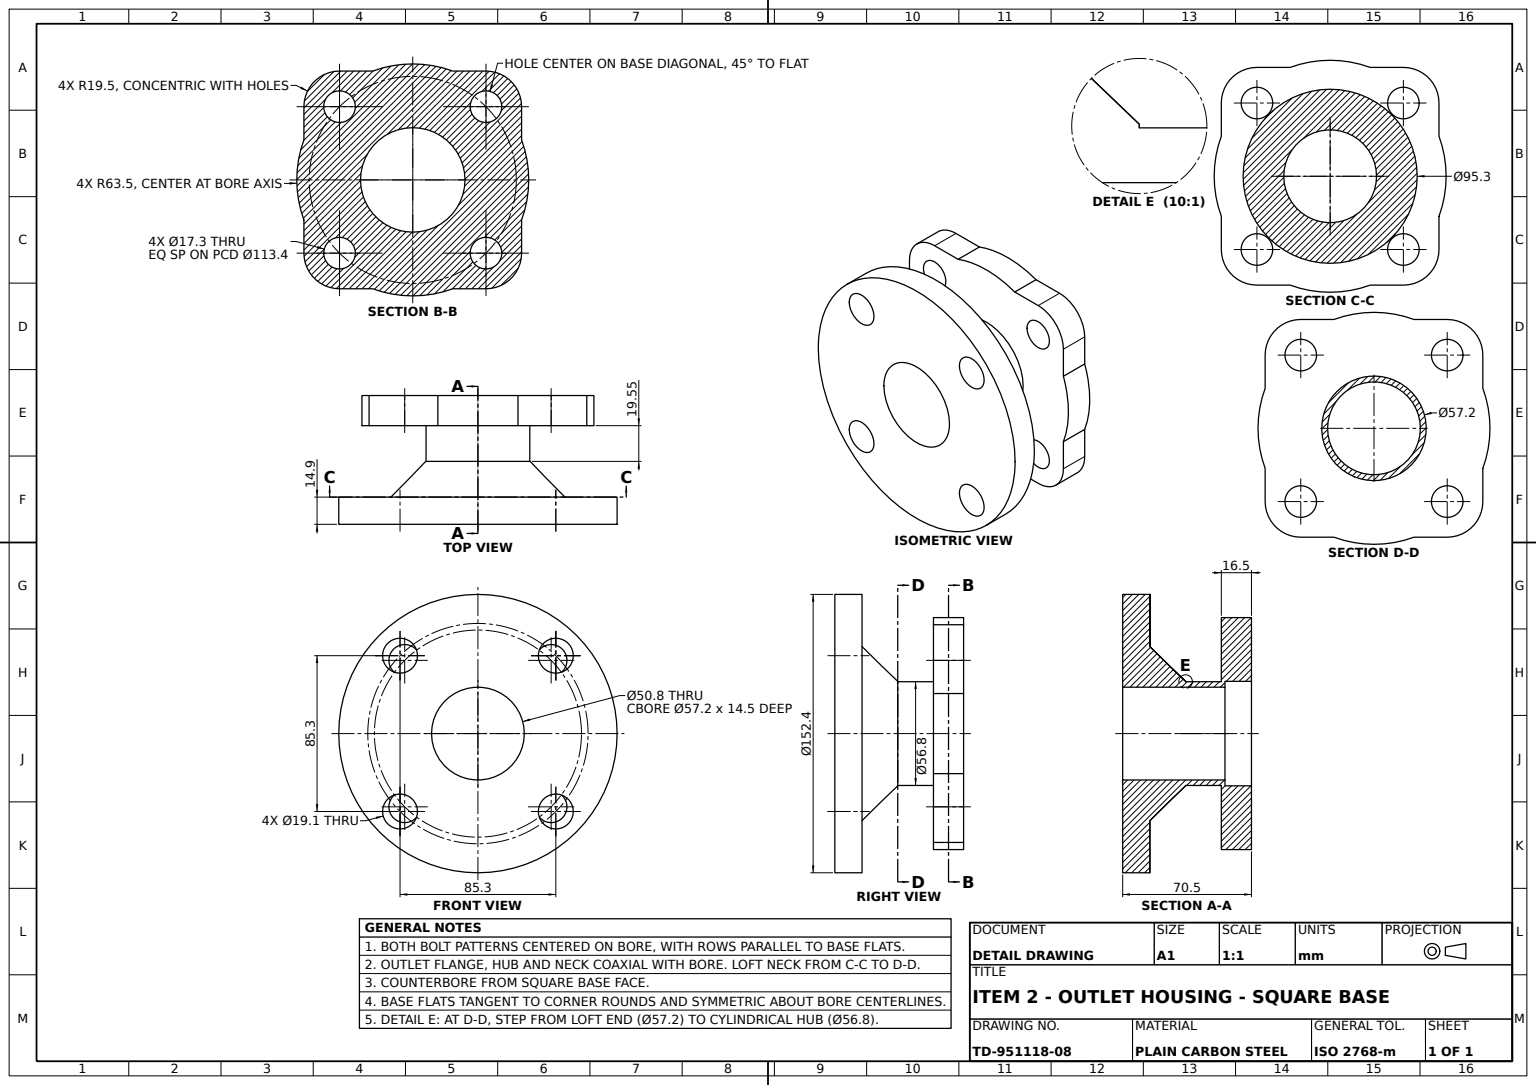
ISO-10303-21;
HEADER;
FILE_DESCRIPTION((''),'2;1');
FILE_NAME('','',(''),(''),'','','');
FILE_SCHEMA(('AUTOMOTIVE_DESIGN'));
ENDSEC;
DATA;
#1=APPLICATION_CONTEXT('');
#2=PRODUCT_CONTEXT('',#1,'mechanical');
#3=PRODUCT('','','',(#2));
#4=PRODUCT_DEFINITION_FORMATION('','',#3);
#5=PRODUCT_DEFINITION_CONTEXT('',#1,'design');
#6=PRODUCT_DEFINITION('','',#4,#5);
#7=PRODUCT_DEFINITION_SHAPE('','',#6);
#8=(LENGTH_UNIT()NAMED_UNIT(*)SI_UNIT(.MILLI.,.METRE.));
#9=(NAMED_UNIT(*)PLANE_ANGLE_UNIT()SI_UNIT($,.RADIAN.));
#10=(NAMED_UNIT(*)SI_UNIT($,.STERADIAN.)SOLID_ANGLE_UNIT());
#11=UNCERTAINTY_MEASURE_WITH_UNIT(LENGTH_MEASURE(1.E-05),#8,'distance_accuracy_value','');
#12=(GEOMETRIC_REPRESENTATION_CONTEXT(3)GLOBAL_UNCERTAINTY_ASSIGNED_CONTEXT((#11))GLOBAL_UNIT_ASSIGNED_CONTEXT((#8,#9,#10))REPRESENTATION_CONTEXT('',''));
#13=CARTESIAN_POINT('',(48.742954,40.092954,16.5));
#14=VERTEX_POINT('',#13);
#15=CARTESIAN_POINT('',(31.442954,40.092954,16.5));
#16=VERTEX_POINT('',#15);
#17=CARTESIAN_POINT('',(40.092954,40.092954,16.5));
#18=DIRECTION('',(0.,0.,1.));
#19=DIRECTION('',(1.,0.,0.));
#20=AXIS2_PLACEMENT_3D('',#17,#18,#19);
#21=CIRCLE('',#20,8.65);
#22=EDGE_CURVE('',#14,#16,#21,.T.);
#23=ORIENTED_EDGE('',*,*,#22,.F.);
#24=EDGE_CURVE('',#16,#14,#21,.T.);
#25=ORIENTED_EDGE('',*,*,#24,.F.);
#26=EDGE_LOOP('',(#23,#25));
#27=FACE_BOUND('',#26,.T.);
#28=CARTESIAN_POINT('',(-31.442954,-40.092954,16.5));
#29=VERTEX_POINT('',#28);
#30=CARTESIAN_POINT('',(-48.742954,-40.092954,16.5));
#31=VERTEX_POINT('',#30);
#32=CARTESIAN_POINT('',(-40.092954,-40.092954,16.5));
#33=AXIS2_PLACEMENT_3D('',#32,#18,#19);
#34=CIRCLE('',#33,8.65);
#35=EDGE_CURVE('',#29,#31,#34,.T.);
#36=ORIENTED_EDGE('',*,*,#35,.F.);
#37=EDGE_CURVE('',#31,#29,#34,.T.);
#38=ORIENTED_EDGE('',*,*,#37,.F.);
#39=EDGE_LOOP('',(#36,#38));
#40=FACE_BOUND('',#39,.T.);
#41=CARTESIAN_POINT('',(-48.742954,40.092954,16.5));
#42=VERTEX_POINT('',#41);
#43=CARTESIAN_POINT('',(-31.442954,40.092954,16.5));
#44=VERTEX_POINT('',#43);
#45=CARTESIAN_POINT('',(-40.092954,40.092954,16.5));
#46=AXIS2_PLACEMENT_3D('',#45,#18,#19);
#47=CIRCLE('',#46,8.65);
#48=EDGE_CURVE('',#42,#44,#47,.T.);
#49=ORIENTED_EDGE('',*,*,#48,.F.);
#50=EDGE_CURVE('',#44,#42,#47,.T.);
#51=ORIENTED_EDGE('',*,*,#50,.F.);
#52=EDGE_LOOP('',(#49,#51));
#53=FACE_BOUND('',#52,.T.);
#54=CARTESIAN_POINT('',(48.742954,-40.092954,16.5));
#55=VERTEX_POINT('',#54);
#56=CARTESIAN_POINT('',(31.442954,-40.092954,16.5));
#57=VERTEX_POINT('',#56);
#58=CARTESIAN_POINT('',(40.092954,-40.092954,16.5));
#59=AXIS2_PLACEMENT_3D('',#58,#18,#19);
#60=CIRCLE('',#59,8.65);
#61=EDGE_CURVE('',#55,#57,#60,.T.);
#62=ORIENTED_EDGE('',*,*,#61,.F.);
#63=EDGE_CURVE('',#57,#55,#60,.T.);
#64=ORIENTED_EDGE('',*,*,#63,.F.);
#65=EDGE_LOOP('',(#62,#64));
#66=FACE_BOUND('',#65,.T.);
#67=CARTESIAN_POINT('',(59.592954,-21.930111,16.5));
#68=VERTEX_POINT('',#67);
#69=CARTESIAN_POINT('',(59.592954,21.930111,16.5));
#70=VERTEX_POINT('',#69);
#71=CARTESIAN_POINT('',(0.,0.,16.5));
#72=AXIS2_PLACEMENT_3D('',#71,#18,#19);
#73=CIRCLE('',#72,63.5);
#74=EDGE_CURVE('',#68,#70,#73,.T.);
#75=ORIENTED_EDGE('',*,*,#74,.T.);
#76=CARTESIAN_POINT('',(59.592954,40.092954,16.5));
#77=VERTEX_POINT('',#76);
#78=CARTESIAN_POINT('',(59.592954,0.,16.5));
#79=DIRECTION('',(0.,1.,0.));
#80=VECTOR('',#79,1000.);
#81=LINE('',#78,#80);
#82=EDGE_CURVE('',#70,#77,#81,.T.);
#83=ORIENTED_EDGE('',*,*,#82,.T.);
#84=CARTESIAN_POINT('',(40.092954,59.592954,16.5));
#85=VERTEX_POINT('',#84);
#86=CIRCLE('',#20,19.5);
#87=EDGE_CURVE('',#77,#85,#86,.T.);
#88=ORIENTED_EDGE('',*,*,#87,.T.);
#89=CARTESIAN_POINT('',(21.930111,59.592954,16.5));
#90=VERTEX_POINT('',#89);
#91=CARTESIAN_POINT('',(0.,59.592954,16.5));
#92=VECTOR('',#19,1000.);
#93=LINE('',#91,#92);
#94=EDGE_CURVE('',#90,#85,#93,.T.);
#95=ORIENTED_EDGE('',*,*,#94,.F.);
#96=CARTESIAN_POINT('',(-21.930111,59.592954,16.5));
#97=VERTEX_POINT('',#96);
#98=EDGE_CURVE('',#90,#97,#73,.T.);
#99=ORIENTED_EDGE('',*,*,#98,.T.);
#100=CARTESIAN_POINT('',(-40.092954,59.592954,16.5));
#101=VERTEX_POINT('',#100);
#102=EDGE_CURVE('',#101,#97,#93,.T.);
#103=ORIENTED_EDGE('',*,*,#102,.F.);
#104=CARTESIAN_POINT('',(-59.592954,40.092954,16.5));
#105=VERTEX_POINT('',#104);
#106=DIRECTION('',(0.,0.,-1.));
#107=AXIS2_PLACEMENT_3D('',#45,#106,#19);
#108=CIRCLE('',#107,19.5);
#109=EDGE_CURVE('',#105,#101,#108,.T.);
#110=ORIENTED_EDGE('',*,*,#109,.F.);
#111=CARTESIAN_POINT('',(-59.592954,21.930111,16.5));
#112=VERTEX_POINT('',#111);
#113=CARTESIAN_POINT('',(-59.592954,0.,16.5));
#114=LINE('',#113,#80);
#115=EDGE_CURVE('',#112,#105,#114,.T.);
#116=ORIENTED_EDGE('',*,*,#115,.F.);
#117=CARTESIAN_POINT('',(-63.5,0.,16.5));
#118=VERTEX_POINT('',#117);
#119=EDGE_CURVE('',#112,#118,#73,.T.);
#120=ORIENTED_EDGE('',*,*,#119,.T.);
#121=CARTESIAN_POINT('',(-59.592954,-21.930111,16.5));
#122=VERTEX_POINT('',#121);
#123=EDGE_CURVE('',#118,#122,#73,.T.);
#124=ORIENTED_EDGE('',*,*,#123,.T.);
#125=CARTESIAN_POINT('',(-59.592954,-40.092954,16.5));
#126=VERTEX_POINT('',#125);
#127=EDGE_CURVE('',#126,#122,#114,.T.);
#128=ORIENTED_EDGE('',*,*,#127,.F.);
#129=CARTESIAN_POINT('',(-40.092954,-59.592954,16.5));
#130=VERTEX_POINT('',#129);
#131=CIRCLE('',#33,19.5);
#132=EDGE_CURVE('',#126,#130,#131,.T.);
#133=ORIENTED_EDGE('',*,*,#132,.T.);
#134=CARTESIAN_POINT('',(-21.930111,-59.592954,16.5));
#135=VERTEX_POINT('',#134);
#136=CARTESIAN_POINT('',(0.,-59.592954,16.5));
#137=DIRECTION('',(-1.,0.,0.));
#138=VECTOR('',#137,1000.);
#139=LINE('',#136,#138);
#140=EDGE_CURVE('',#135,#130,#139,.T.);
#141=ORIENTED_EDGE('',*,*,#140,.F.);
#142=CARTESIAN_POINT('',(21.930111,-59.592954,16.5));
#143=VERTEX_POINT('',#142);
#144=EDGE_CURVE('',#135,#143,#73,.T.);
#145=ORIENTED_EDGE('',*,*,#144,.T.);
#146=CARTESIAN_POINT('',(40.092954,-59.592954,16.5));
#147=VERTEX_POINT('',#146);
#148=EDGE_CURVE('',#147,#143,#139,.T.);
#149=ORIENTED_EDGE('',*,*,#148,.F.);
#150=CARTESIAN_POINT('',(59.592954,-40.092954,16.5));
#151=VERTEX_POINT('',#150);
#152=AXIS2_PLACEMENT_3D('',#58,#106,#19);
#153=CIRCLE('',#152,19.5);
#154=EDGE_CURVE('',#151,#147,#153,.T.);
#155=ORIENTED_EDGE('',*,*,#154,.F.);
#156=DIRECTION('',(0.,-1.,0.));
#157=VECTOR('',#156,1000.);
#158=LINE('',#78,#157);
#159=EDGE_CURVE('',#68,#151,#158,.T.);
#160=ORIENTED_EDGE('',*,*,#159,.F.);
#161=EDGE_LOOP('',(#75,#83,#88,#95,#99,#103,#110,#116,#120,#124,#128,#133,#141,#145,#149,#155,#160));
#162=FACE_OUTER_BOUND('',#161,.T.);
#163=CARTESIAN_POINT('',(-28.4,0.,16.5));
#164=VERTEX_POINT('',#163);
#165=CARTESIAN_POINT('',(28.4,0.,16.5));
#166=VERTEX_POINT('',#165);
#167=CIRCLE('',#72,28.4);
#168=EDGE_CURVE('',#164,#166,#167,.T.);
#169=ORIENTED_EDGE('',*,*,#168,.F.);
#170=EDGE_CURVE('',#166,#164,#167,.T.);
#171=ORIENTED_EDGE('',*,*,#170,.F.);
#172=EDGE_LOOP('',(#169,#171));
#173=FACE_BOUND('',#172,.T.);
#174=PLANE('',#72);
#175=ADVANCED_FACE('',(#27,#40,#53,#66,#162,#173),#174,.T.);
#176=CARTESIAN_POINT('',(-25.4,0.,14.5));
#177=VERTEX_POINT('',#176);
#178=CARTESIAN_POINT('',(25.4,0.,14.5));
#179=VERTEX_POINT('',#178);
#180=CARTESIAN_POINT('',(0.,0.,14.5));
#181=AXIS2_PLACEMENT_3D('',#180,#106,#137);
#182=CIRCLE('',#181,25.4);
#183=EDGE_CURVE('',#177,#179,#182,.T.);
#184=ORIENTED_EDGE('',*,*,#183,.F.);
#185=EDGE_CURVE('',#179,#177,#182,.T.);
#186=ORIENTED_EDGE('',*,*,#185,.F.);
#187=EDGE_LOOP('',(#184,#186));
#188=FACE_BOUND('',#187,.T.);
#189=CARTESIAN_POINT('',(-28.6,0.,14.5));
#190=VERTEX_POINT('',#189);
#191=CARTESIAN_POINT('',(28.6,0.,14.5));
#192=VERTEX_POINT('',#191);
#193=CIRCLE('',#181,28.6);
#194=EDGE_CURVE('',#190,#192,#193,.T.);
#195=ORIENTED_EDGE('',*,*,#194,.T.);
#196=EDGE_CURVE('',#192,#190,#193,.T.);
#197=ORIENTED_EDGE('',*,*,#196,.T.);
#198=EDGE_LOOP('',(#195,#197));
#199=FACE_OUTER_BOUND('',#198,.T.);
#200=PLANE('',#181);
#201=ADVANCED_FACE('',(#188,#199),#200,.T.);
#202=CARTESIAN_POINT('',(-31.442954,40.092954,0.));
#203=VERTEX_POINT('',#202);
#204=CARTESIAN_POINT('',(-31.442954,40.092954,43.5));
#205=VECTOR('',#106,1000.);
#206=LINE('',#204,#205);
#207=EDGE_CURVE('',#44,#203,#206,.T.);
#208=ORIENTED_EDGE('',*,*,#207,.T.);
#209=CARTESIAN_POINT('',(-48.742954,40.092954,0.));
#210=VERTEX_POINT('',#209);
#211=CARTESIAN_POINT('',(-40.092954,40.092954,0.));
#212=AXIS2_PLACEMENT_3D('',#211,#106,#137);
#213=CIRCLE('',#212,8.65);
#214=EDGE_CURVE('',#203,#210,#213,.T.);
#215=ORIENTED_EDGE('',*,*,#214,.T.);
#216=CARTESIAN_POINT('',(-48.742954,40.092954,43.5));
#217=LINE('',#216,#205);
#218=EDGE_CURVE('',#42,#210,#217,.T.);
#219=ORIENTED_EDGE('',*,*,#218,.F.);
#220=ORIENTED_EDGE('',*,*,#48,.T.);
#221=EDGE_LOOP('',(#208,#215,#219,#220));
#222=FACE_OUTER_BOUND('',#221,.T.);
#223=CARTESIAN_POINT('',(-40.092954,40.092954,43.5));
#224=AXIS2_PLACEMENT_3D('',#223,#106,#137);
#225=CYLINDRICAL_SURFACE('',#224,8.65);
#226=ADVANCED_FACE('',(#222),#225,.F.);
#227=CARTESIAN_POINT('',(25.4,0.,70.5));
#228=VERTEX_POINT('',#227);
#229=CARTESIAN_POINT('',(-25.4,0.,70.5));
#230=VERTEX_POINT('',#229);
#231=CARTESIAN_POINT('',(0.,0.,70.5));
#232=AXIS2_PLACEMENT_3D('',#231,#18,#19);
#233=CIRCLE('',#232,25.4);
#234=EDGE_CURVE('',#228,#230,#233,.T.);
#235=ORIENTED_EDGE('',*,*,#234,.T.);
#236=CARTESIAN_POINT('',(-25.4,0.,109.9));
#237=LINE('',#236,#205);
#238=EDGE_CURVE('',#230,#177,#237,.T.);
#239=ORIENTED_EDGE('',*,*,#238,.T.);
#240=ORIENTED_EDGE('',*,*,#183,.T.);
#241=CARTESIAN_POINT('',(25.4,0.,109.9));
#242=LINE('',#241,#205);
#243=EDGE_CURVE('',#228,#179,#242,.T.);
#244=ORIENTED_EDGE('',*,*,#243,.F.);
#245=EDGE_LOOP('',(#235,#239,#240,#244));
#246=FACE_OUTER_BOUND('',#245,.T.);
#247=CARTESIAN_POINT('',(0.,0.,109.9));
#248=AXIS2_PLACEMENT_3D('',#247,#106,#137);
#249=CYLINDRICAL_SURFACE('',#248,25.4);
#250=ADVANCED_FACE('',(#246),#249,.F.);
#251=CARTESIAN_POINT('',(-40.092954,-59.592954,0.));
#252=VERTEX_POINT('',#251);
#253=LINE('',#129,#205);
#254=EDGE_CURVE('',#130,#252,#253,.T.);
#255=ORIENTED_EDGE('',*,*,#254,.T.);
#256=CARTESIAN_POINT('',(-21.930111,-59.592954,0.));
#257=VERTEX_POINT('',#256);
#258=CARTESIAN_POINT('',(0.,-59.592954,0.));
#259=LINE('',#258,#138);
#260=EDGE_CURVE('',#257,#252,#259,.T.);
#261=ORIENTED_EDGE('',*,*,#260,.F.);
#262=LINE('',#134,#205);
#263=EDGE_CURVE('',#135,#257,#262,.T.);
#264=ORIENTED_EDGE('',*,*,#263,.F.);
#265=ORIENTED_EDGE('',*,*,#140,.T.);
#266=EDGE_LOOP('',(#255,#261,#264,#265));
#267=FACE_OUTER_BOUND('',#266,.T.);
#268=AXIS2_PLACEMENT_3D('',#136,#156,#106);
#269=PLANE('',#268);
#270=ADVANCED_FACE('',(#267),#269,.T.);
#271=CARTESIAN_POINT('',(33.1,42.65,55.6));
#272=VERTEX_POINT('',#271);
#273=CARTESIAN_POINT('',(33.1,42.65,70.5));
#274=VERTEX_POINT('',#273);
#275=CARTESIAN_POINT('',(33.1,42.65,34.6));
#276=VECTOR('',#18,1000.);
#277=LINE('',#275,#276);
#278=EDGE_CURVE('',#272,#274,#277,.T.);
#279=ORIENTED_EDGE('',*,*,#278,.F.);
#280=CARTESIAN_POINT('',(52.2,42.65,55.6));
#281=VERTEX_POINT('',#280);
#282=CARTESIAN_POINT('',(42.65,42.65,55.6));
#283=AXIS2_PLACEMENT_3D('',#282,#18,#19);
#284=CIRCLE('',#283,9.55);
#285=EDGE_CURVE('',#281,#272,#284,.T.);
#286=ORIENTED_EDGE('',*,*,#285,.F.);
#287=CARTESIAN_POINT('',(52.2,42.65,70.5));
#288=VERTEX_POINT('',#287);
#289=CARTESIAN_POINT('',(52.2,42.65,34.6));
#290=LINE('',#289,#276);
#291=EDGE_CURVE('',#281,#288,#290,.T.);
#292=ORIENTED_EDGE('',*,*,#291,.T.);
#293=CARTESIAN_POINT('',(42.65,42.65,70.5));
#294=AXIS2_PLACEMENT_3D('',#293,#18,#19);
#295=CIRCLE('',#294,9.55);
#296=EDGE_CURVE('',#288,#274,#295,.T.);
#297=ORIENTED_EDGE('',*,*,#296,.T.);
#298=EDGE_LOOP('',(#279,#286,#292,#297));
#299=FACE_OUTER_BOUND('',#298,.T.);
#300=CARTESIAN_POINT('',(42.65,42.65,34.6));
#301=AXIS2_PLACEMENT_3D('',#300,#18,#19);
#302=CYLINDRICAL_SURFACE('',#301,9.55);
#303=ADVANCED_FACE('',(#299),#302,.F.);
#304=EDGE_CURVE('',#274,#288,#295,.T.);
#305=ORIENTED_EDGE('',*,*,#304,.T.);
#306=ORIENTED_EDGE('',*,*,#291,.F.);
#307=EDGE_CURVE('',#272,#281,#284,.T.);
#308=ORIENTED_EDGE('',*,*,#307,.F.);
#309=ORIENTED_EDGE('',*,*,#278,.T.);
#310=EDGE_LOOP('',(#305,#306,#308,#309));
#311=FACE_OUTER_BOUND('',#310,.T.);
#312=ADVANCED_FACE('',(#311),#302,.F.);
#313=CARTESIAN_POINT('',(-52.2,-42.65,55.6));
#314=VERTEX_POINT('',#313);
#315=CARTESIAN_POINT('',(-52.2,-42.65,70.5));
#316=VERTEX_POINT('',#315);
#317=CARTESIAN_POINT('',(-52.2,-42.65,34.6));
#318=LINE('',#317,#276);
#319=EDGE_CURVE('',#314,#316,#318,.T.);
#320=ORIENTED_EDGE('',*,*,#319,.F.);
#321=CARTESIAN_POINT('',(-33.1,-42.65,55.6));
#322=VERTEX_POINT('',#321);
#323=CARTESIAN_POINT('',(-42.65,-42.65,55.6));
#324=AXIS2_PLACEMENT_3D('',#323,#18,#19);
#325=CIRCLE('',#324,9.55);
#326=EDGE_CURVE('',#322,#314,#325,.T.);
#327=ORIENTED_EDGE('',*,*,#326,.F.);
#328=CARTESIAN_POINT('',(-33.1,-42.65,70.5));
#329=VERTEX_POINT('',#328);
#330=CARTESIAN_POINT('',(-33.1,-42.65,34.6));
#331=LINE('',#330,#276);
#332=EDGE_CURVE('',#322,#329,#331,.T.);
#333=ORIENTED_EDGE('',*,*,#332,.T.);
#334=CARTESIAN_POINT('',(-42.65,-42.65,70.5));
#335=AXIS2_PLACEMENT_3D('',#334,#18,#19);
#336=CIRCLE('',#335,9.55);
#337=EDGE_CURVE('',#329,#316,#336,.T.);
#338=ORIENTED_EDGE('',*,*,#337,.T.);
#339=EDGE_LOOP('',(#320,#327,#333,#338));
#340=FACE_OUTER_BOUND('',#339,.T.);
#341=CARTESIAN_POINT('',(-42.65,-42.65,34.6));
#342=AXIS2_PLACEMENT_3D('',#341,#18,#19);
#343=CYLINDRICAL_SURFACE('',#342,9.55);
#344=ADVANCED_FACE('',(#340),#343,.F.);
#345=CARTESIAN_POINT('',(59.592954,21.930111,0.));
#346=VERTEX_POINT('',#345);
#347=CARTESIAN_POINT('',(59.592954,40.092954,0.));
#348=VERTEX_POINT('',#347);
#349=CARTESIAN_POINT('',(59.592954,0.,0.));
#350=LINE('',#349,#80);
#351=EDGE_CURVE('',#346,#348,#350,.T.);
#352=ORIENTED_EDGE('',*,*,#351,.T.);
#353=LINE('',#76,#205);
#354=EDGE_CURVE('',#77,#348,#353,.T.);
#355=ORIENTED_EDGE('',*,*,#354,.F.);
#356=ORIENTED_EDGE('',*,*,#82,.F.);
#357=LINE('',#69,#205);
#358=EDGE_CURVE('',#70,#346,#357,.T.);
#359=ORIENTED_EDGE('',*,*,#358,.T.);
#360=EDGE_LOOP('',(#352,#355,#356,#359));
#361=FACE_OUTER_BOUND('',#360,.T.);
#362=AXIS2_PLACEMENT_3D('',#78,#137,#18);
#363=PLANE('',#362);
#364=ADVANCED_FACE('',(#361),#363,.F.);
#365=CARTESIAN_POINT('',(40.092954,59.592954,0.));
#366=VERTEX_POINT('',#365);
#367=LINE('',#84,#205);
#368=EDGE_CURVE('',#85,#366,#367,.T.);
#369=ORIENTED_EDGE('',*,*,#368,.F.);
#370=ORIENTED_EDGE('',*,*,#87,.F.);
#371=ORIENTED_EDGE('',*,*,#354,.T.);
#372=CARTESIAN_POINT('',(40.092954,40.092954,0.));
#373=AXIS2_PLACEMENT_3D('',#372,#18,#19);
#374=CIRCLE('',#373,19.5);
#375=EDGE_CURVE('',#348,#366,#374,.T.);
#376=ORIENTED_EDGE('',*,*,#375,.T.);
#377=EDGE_LOOP('',(#369,#370,#371,#376));
#378=FACE_OUTER_BOUND('',#377,.T.);
#379=AXIS2_PLACEMENT_3D('',#17,#106,#137);
#380=CYLINDRICAL_SURFACE('',#379,19.5);
#381=ADVANCED_FACE('',(#378),#380,.T.);
#382=ORIENTED_EDGE('',*,*,#132,.F.);
#383=CARTESIAN_POINT('',(-59.592954,-40.092954,0.));
#384=VERTEX_POINT('',#383);
#385=LINE('',#125,#205);
#386=EDGE_CURVE('',#126,#384,#385,.T.);
#387=ORIENTED_EDGE('',*,*,#386,.T.);
#388=CARTESIAN_POINT('',(-40.092954,-40.092954,0.));
#389=AXIS2_PLACEMENT_3D('',#388,#18,#19);
#390=CIRCLE('',#389,19.5);
#391=EDGE_CURVE('',#384,#252,#390,.T.);
#392=ORIENTED_EDGE('',*,*,#391,.T.);
#393=ORIENTED_EDGE('',*,*,#254,.F.);
#394=EDGE_LOOP('',(#382,#387,#392,#393));
#395=FACE_OUTER_BOUND('',#394,.T.);
#396=AXIS2_PLACEMENT_3D('',#32,#106,#137);
#397=CYLINDRICAL_SURFACE('',#396,19.5);
#398=ADVANCED_FACE('',(#395),#397,.T.);
#399=CARTESIAN_POINT('',(52.2,-42.65,55.6));
#400=VERTEX_POINT('',#399);
#401=CARTESIAN_POINT('',(52.2,-42.65,70.5));
#402=VERTEX_POINT('',#401);
#403=CARTESIAN_POINT('',(52.2,-42.65,34.6));
#404=LINE('',#403,#276);
#405=EDGE_CURVE('',#400,#402,#404,.T.);
#406=ORIENTED_EDGE('',*,*,#405,.F.);
#407=CARTESIAN_POINT('',(33.1,-42.65,55.6));
#408=VERTEX_POINT('',#407);
#409=CARTESIAN_POINT('',(42.65,-42.65,55.6));
#410=AXIS2_PLACEMENT_3D('',#409,#18,#19);
#411=CIRCLE('',#410,9.55);
#412=EDGE_CURVE('',#408,#400,#411,.T.);
#413=ORIENTED_EDGE('',*,*,#412,.F.);
#414=CARTESIAN_POINT('',(33.1,-42.65,70.5));
#415=VERTEX_POINT('',#414);
#416=CARTESIAN_POINT('',(33.1,-42.65,34.6));
#417=LINE('',#416,#276);
#418=EDGE_CURVE('',#408,#415,#417,.T.);
#419=ORIENTED_EDGE('',*,*,#418,.T.);
#420=CARTESIAN_POINT('',(42.65,-42.65,70.5));
#421=AXIS2_PLACEMENT_3D('',#420,#18,#19);
#422=CIRCLE('',#421,9.55);
#423=EDGE_CURVE('',#415,#402,#422,.T.);
#424=ORIENTED_EDGE('',*,*,#423,.T.);
#425=EDGE_LOOP('',(#406,#413,#419,#424));
#426=FACE_OUTER_BOUND('',#425,.T.);
#427=CARTESIAN_POINT('',(42.65,-42.65,34.6));
#428=AXIS2_PLACEMENT_3D('',#427,#18,#19);
#429=CYLINDRICAL_SURFACE('',#428,9.55);
#430=ADVANCED_FACE('',(#426),#429,.F.);
#431=ORIENTED_EDGE('',*,*,#74,.F.);
#432=CARTESIAN_POINT('',(59.592954,-21.930111,0.));
#433=VERTEX_POINT('',#432);
#434=LINE('',#67,#205);
#435=EDGE_CURVE('',#68,#433,#434,.T.);
#436=ORIENTED_EDGE('',*,*,#435,.T.);
#437=CARTESIAN_POINT('',(0.,0.,0.));
#438=AXIS2_PLACEMENT_3D('',#437,#18,#19);
#439=CIRCLE('',#438,63.5);
#440=EDGE_CURVE('',#433,#346,#439,.T.);
#441=ORIENTED_EDGE('',*,*,#440,.T.);
#442=ORIENTED_EDGE('',*,*,#358,.F.);
#443=EDGE_LOOP('',(#431,#436,#441,#442));
#444=FACE_OUTER_BOUND('',#443,.T.);
#445=AXIS2_PLACEMENT_3D('',#71,#106,#137);
#446=CYLINDRICAL_SURFACE('',#445,63.5);
#447=ADVANCED_FACE('',(#444),#446,.T.);
#448=CARTESIAN_POINT('',(-48.742954,-40.092954,0.));
#449=VERTEX_POINT('',#448);
#450=CARTESIAN_POINT('',(-48.742954,-40.092954,43.5));
#451=LINE('',#450,#205);
#452=EDGE_CURVE('',#31,#449,#451,.T.);
#453=ORIENTED_EDGE('',*,*,#452,.T.);
#454=CARTESIAN_POINT('',(-31.442954,-40.092954,0.));
#455=VERTEX_POINT('',#454);
#456=AXIS2_PLACEMENT_3D('',#388,#106,#19);
#457=CIRCLE('',#456,8.65);
#458=EDGE_CURVE('',#449,#455,#457,.T.);
#459=ORIENTED_EDGE('',*,*,#458,.T.);
#460=CARTESIAN_POINT('',(-31.442954,-40.092954,43.5));
#461=LINE('',#460,#205);
#462=EDGE_CURVE('',#29,#455,#461,.T.);
#463=ORIENTED_EDGE('',*,*,#462,.F.);
#464=ORIENTED_EDGE('',*,*,#35,.T.);
#465=EDGE_LOOP('',(#453,#459,#463,#464));
#466=FACE_OUTER_BOUND('',#465,.T.);
#467=CARTESIAN_POINT('',(-40.092954,-40.092954,43.5));
#468=AXIS2_PLACEMENT_3D('',#467,#106,#137);
#469=CYLINDRICAL_SURFACE('',#468,8.65);
#470=ADVANCED_FACE('',(#466),#469,.F.);
#471=CARTESIAN_POINT('',(-28.6,0.,0.));
#472=VERTEX_POINT('',#471);
#473=CARTESIAN_POINT('',(28.6,0.,0.));
#474=VERTEX_POINT('',#473);
#475=CIRCLE('',#438,28.6);
#476=EDGE_CURVE('',#472,#474,#475,.T.);
#477=ORIENTED_EDGE('',*,*,#476,.F.);
#478=CARTESIAN_POINT('',(-28.6,0.,-27.));
#479=LINE('',#478,#276);
#480=EDGE_CURVE('',#472,#190,#479,.T.);
#481=ORIENTED_EDGE('',*,*,#480,.T.);
#482=ORIENTED_EDGE('',*,*,#196,.F.);
#483=CARTESIAN_POINT('',(28.6,0.,-27.));
#484=LINE('',#483,#276);
#485=EDGE_CURVE('',#474,#192,#484,.T.);
#486=ORIENTED_EDGE('',*,*,#485,.F.);
#487=EDGE_LOOP('',(#477,#481,#482,#486));
#488=FACE_OUTER_BOUND('',#487,.T.);
#489=CARTESIAN_POINT('',(0.,0.,-27.));
#490=AXIS2_PLACEMENT_3D('',#489,#18,#19);
#491=CYLINDRICAL_SURFACE('',#490,28.6);
#492=ADVANCED_FACE('',(#488),#491,.F.);
#493=CARTESIAN_POINT('',(-33.1,42.65,55.6));
#494=VERTEX_POINT('',#493);
#495=CARTESIAN_POINT('',(-33.1,42.65,70.5));
#496=VERTEX_POINT('',#495);
#497=CARTESIAN_POINT('',(-33.1,42.65,34.6));
#498=LINE('',#497,#276);
#499=EDGE_CURVE('',#494,#496,#498,.T.);
#500=ORIENTED_EDGE('',*,*,#499,.T.);
#501=CARTESIAN_POINT('',(-52.2,42.65,70.5));
#502=VERTEX_POINT('',#501);
#503=CARTESIAN_POINT('',(-42.65,42.65,70.5));
#504=AXIS2_PLACEMENT_3D('',#503,#18,#19);
#505=CIRCLE('',#504,9.55);
#506=EDGE_CURVE('',#496,#502,#505,.T.);
#507=ORIENTED_EDGE('',*,*,#506,.T.);
#508=CARTESIAN_POINT('',(-52.2,42.65,55.6));
#509=VERTEX_POINT('',#508);
#510=CARTESIAN_POINT('',(-52.2,42.65,34.6));
#511=LINE('',#510,#276);
#512=EDGE_CURVE('',#509,#502,#511,.T.);
#513=ORIENTED_EDGE('',*,*,#512,.F.);
#514=CARTESIAN_POINT('',(-42.65,42.65,55.6));
#515=AXIS2_PLACEMENT_3D('',#514,#18,#19);
#516=CIRCLE('',#515,9.55);
#517=EDGE_CURVE('',#494,#509,#516,.T.);
#518=ORIENTED_EDGE('',*,*,#517,.F.);
#519=EDGE_LOOP('',(#500,#507,#513,#518));
#520=FACE_OUTER_BOUND('',#519,.T.);
#521=CARTESIAN_POINT('',(-42.65,42.65,34.6));
#522=AXIS2_PLACEMENT_3D('',#521,#18,#19);
#523=CYLINDRICAL_SURFACE('',#522,9.55);
#524=ADVANCED_FACE('',(#520),#523,.F.);
#525=CARTESIAN_POINT('',(-10.645216,-26.545044,36.05));
#526=VERTEX_POINT('',#525);
#527=CARTESIAN_POINT('',(-25.329596,-40.360056,55.6));
#528=VERTEX_POINT('',#527);
#529=B_SPLINE_CURVE_WITH_KNOTS('',1,(#525,#527),.UNSPECIFIED.,.F.,.F.,(2,2),(0.,1.),.UNSPECIFIED.);
#530=EDGE_CURVE('',#526,#528,#529,.T.);
#531=ORIENTED_EDGE('',*,*,#530,.T.);
#532=CARTESIAN_POINT('',(25.329596,40.360056,55.6));
#533=VERTEX_POINT('',#532);
#534=CARTESIAN_POINT('',(0.,0.,55.6));
#535=AXIS2_PLACEMENT_3D('',#534,#18,#19);
#536=CIRCLE('',#535,47.65);
#537=EDGE_CURVE('',#533,#528,#536,.T.);
#538=ORIENTED_EDGE('',*,*,#537,.F.);
#539=CARTESIAN_POINT('',(10.645216,26.545044,36.05));
#540=VERTEX_POINT('',#539);
#541=B_SPLINE_CURVE_WITH_KNOTS('',1,(#539,#532),.UNSPECIFIED.,.F.,.F.,(2,2),(0.,1.),.UNSPECIFIED.);
#542=EDGE_CURVE('',#540,#533,#541,.T.);
#543=ORIENTED_EDGE('',*,*,#542,.F.);
#544=CARTESIAN_POINT('',(0.,0.,36.05));
#545=AXIS2_PLACEMENT_3D('',#544,#18,#19);
#546=CIRCLE('',#545,28.6);
#547=EDGE_CURVE('',#540,#526,#546,.T.);
#548=ORIENTED_EDGE('',*,*,#547,.T.);
#549=EDGE_LOOP('',(#531,#538,#543,#548));
#550=FACE_OUTER_BOUND('',#549,.T.);
#551=CARTESIAN_POINT('',(25.329596,40.360055,55.6));
#552=CARTESIAN_POINT('',(-42.444873,47.835476,36.05));
#553=CARTESIAN_POINT('',(-55.390515,91.019247,55.6));
#554=CARTESIAN_POINT('',(-63.735305,-5.254612,36.05));
#555=CARTESIAN_POINT('',(-106.049707,10.299136,55.6));
#556=CARTESIAN_POINT('',(-25.329596,-40.360055,55.6));
#557=CARTESIAN_POINT('',(42.444873,-47.835476,36.05));
#558=CARTESIAN_POINT('',(55.390515,-91.019247,55.6));
#559=CARTESIAN_POINT('',(63.735305,5.254612,36.05));
#560=CARTESIAN_POINT('',(106.049707,-10.299136,55.6));
#561=(BOUNDED_SURFACE()B_SPLINE_SURFACE(3,1,((#539,#551),(#552,#553),(#554,#555),(#525,#556),(#557,#558),(#559,#560),(#539,#551)),.UNSPECIFIED.,.T.,.F.,.F.)B_SPLINE_SURFACE_WITH_KNOTS((4,3,4),(2,2),(0.,0.5,1.),(0.,1.),.UNSPECIFIED.)GEOMETRIC_REPRESENTATION_ITEM()RATIONAL_B_SPLINE_SURFACE(((1.,1.),(0.333333333,0.333333333),(0.333333333,0.333333333),(1.,1.),(0.333333333,0.333333333),(0.333333333,0.333333333),(1.,1.)))REPRESENTATION_ITEM('')SURFACE());
#562=ADVANCED_FACE('',(#550),#561,.T.);
#563=CARTESIAN_POINT('',(-28.4,0.,36.05));
#564=VERTEX_POINT('',#563);
#565=LINE('',#563,#205);
#566=EDGE_CURVE('',#564,#164,#565,.T.);
#567=ORIENTED_EDGE('',*,*,#566,.T.);
#568=ORIENTED_EDGE('',*,*,#168,.T.);
#569=CARTESIAN_POINT('',(28.4,0.,36.05));
#570=VERTEX_POINT('',#569);
#571=LINE('',#569,#205);
#572=EDGE_CURVE('',#570,#166,#571,.T.);
#573=ORIENTED_EDGE('',*,*,#572,.F.);
#574=CIRCLE('',#545,28.4);
#575=EDGE_CURVE('',#564,#570,#574,.T.);
#576=ORIENTED_EDGE('',*,*,#575,.F.);
#577=EDGE_LOOP('',(#567,#568,#573,#576));
#578=FACE_OUTER_BOUND('',#577,.T.);
#579=AXIS2_PLACEMENT_3D('',#544,#106,#137);
#580=CYLINDRICAL_SURFACE('',#579,28.4);
#581=ADVANCED_FACE('',(#578),#580,.T.);
#582=CARTESIAN_POINT('',(-40.092954,59.592954,0.));
#583=VERTEX_POINT('',#582);
#584=LINE('',#100,#205);
#585=EDGE_CURVE('',#101,#583,#584,.T.);
#586=ORIENTED_EDGE('',*,*,#585,.T.);
#587=CARTESIAN_POINT('',(-59.592954,40.092954,0.));
#588=VERTEX_POINT('',#587);
#589=AXIS2_PLACEMENT_3D('',#211,#106,#19);
#590=CIRCLE('',#589,19.5);
#591=EDGE_CURVE('',#588,#583,#590,.T.);
#592=ORIENTED_EDGE('',*,*,#591,.F.);
#593=LINE('',#104,#205);
#594=EDGE_CURVE('',#105,#588,#593,.T.);
#595=ORIENTED_EDGE('',*,*,#594,.F.);
#596=ORIENTED_EDGE('',*,*,#109,.T.);
#597=EDGE_LOOP('',(#586,#592,#595,#596));
#598=FACE_OUTER_BOUND('',#597,.T.);
#599=AXIS2_PLACEMENT_3D('',#45,#106,#137);
#600=CYLINDRICAL_SURFACE('',#599,19.5);
#601=ADVANCED_FACE('',(#598),#600,.T.);
#602=ORIENTED_EDGE('',*,*,#476,.T.);
#603=EDGE_CURVE('',#474,#472,#475,.T.);
#604=ORIENTED_EDGE('',*,*,#603,.T.);
#605=EDGE_LOOP('',(#602,#604));
#606=FACE_BOUND('',#605,.T.);
#607=CARTESIAN_POINT('',(59.592954,-40.092954,0.));
#608=VERTEX_POINT('',#607);
#609=CARTESIAN_POINT('',(40.092954,-59.592954,0.));
#610=VERTEX_POINT('',#609);
#611=CARTESIAN_POINT('',(40.092954,-40.092954,0.));
#612=AXIS2_PLACEMENT_3D('',#611,#106,#19);
#613=CIRCLE('',#612,19.5);
#614=EDGE_CURVE('',#608,#610,#613,.T.);
#615=ORIENTED_EDGE('',*,*,#614,.T.);
#616=CARTESIAN_POINT('',(21.930111,-59.592954,0.));
#617=VERTEX_POINT('',#616);
#618=EDGE_CURVE('',#610,#617,#259,.T.);
#619=ORIENTED_EDGE('',*,*,#618,.T.);
#620=EDGE_CURVE('',#257,#617,#439,.T.);
#621=ORIENTED_EDGE('',*,*,#620,.F.);
#622=ORIENTED_EDGE('',*,*,#260,.T.);
#623=ORIENTED_EDGE('',*,*,#391,.F.);
#624=CARTESIAN_POINT('',(-59.592954,-21.930111,0.));
#625=VERTEX_POINT('',#624);
#626=CARTESIAN_POINT('',(-59.592954,0.,0.));
#627=LINE('',#626,#80);
#628=EDGE_CURVE('',#384,#625,#627,.T.);
#629=ORIENTED_EDGE('',*,*,#628,.T.);
#630=CARTESIAN_POINT('',(-63.5,0.,0.));
#631=VERTEX_POINT('',#630);
#632=EDGE_CURVE('',#631,#625,#439,.T.);
#633=ORIENTED_EDGE('',*,*,#632,.F.);
#634=CARTESIAN_POINT('',(-59.592954,21.930111,0.));
#635=VERTEX_POINT('',#634);
#636=EDGE_CURVE('',#635,#631,#439,.T.);
#637=ORIENTED_EDGE('',*,*,#636,.F.);
#638=EDGE_CURVE('',#635,#588,#627,.T.);
#639=ORIENTED_EDGE('',*,*,#638,.T.);
#640=ORIENTED_EDGE('',*,*,#591,.T.);
#641=CARTESIAN_POINT('',(-21.930111,59.592954,0.));
#642=VERTEX_POINT('',#641);
#643=CARTESIAN_POINT('',(0.,59.592954,0.));
#644=LINE('',#643,#92);
#645=EDGE_CURVE('',#583,#642,#644,.T.);
#646=ORIENTED_EDGE('',*,*,#645,.T.);
#647=CARTESIAN_POINT('',(21.930111,59.592954,0.));
#648=VERTEX_POINT('',#647);
#649=EDGE_CURVE('',#648,#642,#439,.T.);
#650=ORIENTED_EDGE('',*,*,#649,.F.);
#651=EDGE_CURVE('',#648,#366,#644,.T.);
#652=ORIENTED_EDGE('',*,*,#651,.T.);
#653=ORIENTED_EDGE('',*,*,#375,.F.);
#654=ORIENTED_EDGE('',*,*,#351,.F.);
#655=ORIENTED_EDGE('',*,*,#440,.F.);
#656=LINE('',#349,#157);
#657=EDGE_CURVE('',#433,#608,#656,.T.);
#658=ORIENTED_EDGE('',*,*,#657,.T.);
#659=EDGE_LOOP('',(#615,#619,#621,#622,#623,#629,#633,#637,#639,#640,#646,#650,#652,#653,#654,#655,#658));
#660=FACE_OUTER_BOUND('',#659,.T.);
#661=CARTESIAN_POINT('',(48.742954,40.092954,0.));
#662=VERTEX_POINT('',#661);
#663=CARTESIAN_POINT('',(31.442954,40.092954,0.));
#664=VERTEX_POINT('',#663);
#665=AXIS2_PLACEMENT_3D('',#372,#106,#19);
#666=CIRCLE('',#665,8.65);
#667=EDGE_CURVE('',#662,#664,#666,.T.);
#668=ORIENTED_EDGE('',*,*,#667,.F.);
#669=EDGE_CURVE('',#664,#662,#666,.T.);
#670=ORIENTED_EDGE('',*,*,#669,.F.);
#671=EDGE_LOOP('',(#668,#670));
#672=FACE_BOUND('',#671,.T.);
#673=EDGE_CURVE('',#455,#449,#457,.T.);
#674=ORIENTED_EDGE('',*,*,#673,.F.);
#675=ORIENTED_EDGE('',*,*,#458,.F.);
#676=EDGE_LOOP('',(#674,#675));
#677=FACE_BOUND('',#676,.T.);
#678=EDGE_CURVE('',#210,#203,#213,.T.);
#679=ORIENTED_EDGE('',*,*,#678,.F.);
#680=ORIENTED_EDGE('',*,*,#214,.F.);
#681=EDGE_LOOP('',(#679,#680));
#682=FACE_BOUND('',#681,.T.);
#683=CARTESIAN_POINT('',(31.442954,-40.092954,0.));
#684=VERTEX_POINT('',#683);
#685=CARTESIAN_POINT('',(48.742954,-40.092954,0.));
#686=VERTEX_POINT('',#685);
#687=AXIS2_PLACEMENT_3D('',#611,#106,#137);
#688=CIRCLE('',#687,8.65);
#689=EDGE_CURVE('',#684,#686,#688,.T.);
#690=ORIENTED_EDGE('',*,*,#689,.F.);
#691=EDGE_CURVE('',#686,#684,#688,.T.);
#692=ORIENTED_EDGE('',*,*,#691,.F.);
#693=EDGE_LOOP('',(#690,#692));
#694=FACE_BOUND('',#693,.T.);
#695=PLANE('',#438);
#696=ADVANCED_FACE('',(#606,#660,#672,#677,#682,#694),#695,.F.);
#697=ORIENTED_EDGE('',*,*,#123,.F.);
#698=LINE('',#117,#205);
#699=EDGE_CURVE('',#118,#631,#698,.T.);
#700=ORIENTED_EDGE('',*,*,#699,.T.);
#701=ORIENTED_EDGE('',*,*,#632,.T.);
#702=LINE('',#121,#205);
#703=EDGE_CURVE('',#122,#625,#702,.T.);
#704=ORIENTED_EDGE('',*,*,#703,.F.);
#705=EDGE_LOOP('',(#697,#700,#701,#704));
#706=FACE_OUTER_BOUND('',#705,.T.);
#707=ADVANCED_FACE('',(#706),#446,.T.);
#708=ORIENTED_EDGE('',*,*,#628,.F.);
#709=ORIENTED_EDGE('',*,*,#386,.F.);
#710=ORIENTED_EDGE('',*,*,#127,.T.);
#711=ORIENTED_EDGE('',*,*,#703,.T.);
#712=EDGE_LOOP('',(#708,#709,#710,#711));
#713=FACE_OUTER_BOUND('',#712,.T.);
#714=AXIS2_PLACEMENT_3D('',#113,#137,#18);
#715=PLANE('',#714);
#716=ADVANCED_FACE('',(#713),#715,.T.);
#717=LINE('',#111,#205);
#718=EDGE_CURVE('',#112,#635,#717,.T.);
#719=ORIENTED_EDGE('',*,*,#718,.F.);
#720=ORIENTED_EDGE('',*,*,#115,.T.);
#721=ORIENTED_EDGE('',*,*,#594,.T.);
#722=ORIENTED_EDGE('',*,*,#638,.F.);
#723=EDGE_LOOP('',(#719,#720,#721,#722));
#724=FACE_OUTER_BOUND('',#723,.T.);
#725=ADVANCED_FACE('',(#724),#715,.T.);
#726=ORIENTED_EDGE('',*,*,#22,.T.);
#727=CARTESIAN_POINT('',(31.442954,40.092954,43.5));
#728=LINE('',#727,#205);
#729=EDGE_CURVE('',#16,#664,#728,.T.);
#730=ORIENTED_EDGE('',*,*,#729,.T.);
#731=ORIENTED_EDGE('',*,*,#669,.T.);
#732=CARTESIAN_POINT('',(48.742954,40.092954,43.5));
#733=LINE('',#732,#205);
#734=EDGE_CURVE('',#14,#662,#733,.T.);
#735=ORIENTED_EDGE('',*,*,#734,.F.);
#736=EDGE_LOOP('',(#726,#730,#731,#735));
#737=FACE_OUTER_BOUND('',#736,.T.);
#738=CARTESIAN_POINT('',(40.092954,40.092954,43.5));
#739=AXIS2_PLACEMENT_3D('',#738,#106,#137);
#740=CYLINDRICAL_SURFACE('',#739,8.65);
#741=ADVANCED_FACE('',(#737),#740,.F.);
#742=ORIENTED_EDGE('',*,*,#319,.T.);
#743=EDGE_CURVE('',#316,#329,#336,.T.);
#744=ORIENTED_EDGE('',*,*,#743,.T.);
#745=ORIENTED_EDGE('',*,*,#332,.F.);
#746=EDGE_CURVE('',#314,#322,#325,.T.);
#747=ORIENTED_EDGE('',*,*,#746,.F.);
#748=EDGE_LOOP('',(#742,#744,#745,#747));
#749=FACE_OUTER_BOUND('',#748,.T.);
#750=ADVANCED_FACE('',(#749),#343,.F.);
#751=ORIENTED_EDGE('',*,*,#499,.F.);
#752=EDGE_CURVE('',#509,#494,#516,.T.);
#753=ORIENTED_EDGE('',*,*,#752,.F.);
#754=ORIENTED_EDGE('',*,*,#512,.T.);
#755=EDGE_CURVE('',#502,#496,#505,.T.);
#756=ORIENTED_EDGE('',*,*,#755,.T.);
#757=EDGE_LOOP('',(#751,#753,#754,#756));
#758=FACE_OUTER_BOUND('',#757,.T.);
#759=ADVANCED_FACE('',(#758),#523,.F.);
#760=LINE('',#96,#205);
#761=EDGE_CURVE('',#97,#642,#760,.T.);
#762=ORIENTED_EDGE('',*,*,#761,.T.);
#763=ORIENTED_EDGE('',*,*,#645,.F.);
#764=ORIENTED_EDGE('',*,*,#585,.F.);
#765=ORIENTED_EDGE('',*,*,#102,.T.);
#766=EDGE_LOOP('',(#762,#763,#764,#765));
#767=FACE_OUTER_BOUND('',#766,.T.);
#768=AXIS2_PLACEMENT_3D('',#91,#79,#18);
#769=PLANE('',#768);
#770=ADVANCED_FACE('',(#767),#769,.T.);
#771=CARTESIAN_POINT('',(76.2,0.,70.5));
#772=VERTEX_POINT('',#771);
#773=CARTESIAN_POINT('',(-76.2,0.,70.5));
#774=VERTEX_POINT('',#773);
#775=CIRCLE('',#232,76.2);
#776=EDGE_CURVE('',#772,#774,#775,.T.);
#777=ORIENTED_EDGE('',*,*,#776,.T.);
#778=EDGE_CURVE('',#774,#772,#775,.T.);
#779=ORIENTED_EDGE('',*,*,#778,.T.);
#780=EDGE_LOOP('',(#777,#779));
#781=FACE_OUTER_BOUND('',#780,.T.);
#782=ORIENTED_EDGE('',*,*,#506,.F.);
#783=ORIENTED_EDGE('',*,*,#755,.F.);
#784=EDGE_LOOP('',(#782,#783));
#785=FACE_BOUND('',#784,.T.);
#786=ORIENTED_EDGE('',*,*,#234,.F.);
#787=EDGE_CURVE('',#230,#228,#233,.T.);
#788=ORIENTED_EDGE('',*,*,#787,.F.);
#789=EDGE_LOOP('',(#786,#788));
#790=FACE_BOUND('',#789,.T.);
#791=ORIENTED_EDGE('',*,*,#337,.F.);
#792=ORIENTED_EDGE('',*,*,#743,.F.);
#793=EDGE_LOOP('',(#791,#792));
#794=FACE_BOUND('',#793,.T.);
#795=ORIENTED_EDGE('',*,*,#296,.F.);
#796=ORIENTED_EDGE('',*,*,#304,.F.);
#797=EDGE_LOOP('',(#795,#796));
#798=FACE_BOUND('',#797,.T.);
#799=EDGE_CURVE('',#402,#415,#422,.T.);
#800=ORIENTED_EDGE('',*,*,#799,.F.);
#801=ORIENTED_EDGE('',*,*,#423,.F.);
#802=EDGE_LOOP('',(#800,#801));
#803=FACE_BOUND('',#802,.T.);
#804=PLANE('',#232);
#805=ADVANCED_FACE('',(#781,#785,#790,#794,#798,#803),#804,.T.);
#806=ORIENTED_EDGE('',*,*,#566,.F.);
#807=EDGE_CURVE('',#570,#564,#574,.T.);
#808=ORIENTED_EDGE('',*,*,#807,.F.);
#809=ORIENTED_EDGE('',*,*,#572,.T.);
#810=ORIENTED_EDGE('',*,*,#170,.T.);
#811=EDGE_LOOP('',(#806,#808,#809,#810));
#812=FACE_OUTER_BOUND('',#811,.T.);
#813=ADVANCED_FACE('',(#812),#580,.T.);
#814=ORIENTED_EDGE('',*,*,#734,.T.);
#815=ORIENTED_EDGE('',*,*,#667,.T.);
#816=ORIENTED_EDGE('',*,*,#729,.F.);
#817=ORIENTED_EDGE('',*,*,#24,.T.);
#818=EDGE_LOOP('',(#814,#815,#816,#817));
#819=FACE_OUTER_BOUND('',#818,.T.);
#820=ADVANCED_FACE('',(#819),#740,.F.);
#821=ORIENTED_EDGE('',*,*,#405,.T.);
#822=ORIENTED_EDGE('',*,*,#799,.T.);
#823=ORIENTED_EDGE('',*,*,#418,.F.);
#824=EDGE_CURVE('',#400,#408,#411,.T.);
#825=ORIENTED_EDGE('',*,*,#824,.F.);
#826=EDGE_LOOP('',(#821,#822,#823,#825));
#827=FACE_OUTER_BOUND('',#826,.T.);
#828=ADVANCED_FACE('',(#827),#429,.F.);
#829=LINE('',#142,#205);
#830=EDGE_CURVE('',#143,#617,#829,.T.);
#831=ORIENTED_EDGE('',*,*,#830,.T.);
#832=ORIENTED_EDGE('',*,*,#618,.F.);
#833=LINE('',#146,#205);
#834=EDGE_CURVE('',#147,#610,#833,.T.);
#835=ORIENTED_EDGE('',*,*,#834,.F.);
#836=ORIENTED_EDGE('',*,*,#148,.T.);
#837=EDGE_LOOP('',(#831,#832,#835,#836));
#838=FACE_OUTER_BOUND('',#837,.T.);
#839=ADVANCED_FACE('',(#838),#269,.T.);
#840=CARTESIAN_POINT('',(48.742954,-40.092954,43.5));
#841=LINE('',#840,#205);
#842=EDGE_CURVE('',#55,#686,#841,.T.);
#843=ORIENTED_EDGE('',*,*,#842,.T.);
#844=ORIENTED_EDGE('',*,*,#691,.T.);
#845=CARTESIAN_POINT('',(31.442954,-40.092954,43.5));
#846=LINE('',#845,#205);
#847=EDGE_CURVE('',#57,#684,#846,.T.);
#848=ORIENTED_EDGE('',*,*,#847,.F.);
#849=ORIENTED_EDGE('',*,*,#63,.T.);
#850=EDGE_LOOP('',(#843,#844,#848,#849));
#851=FACE_OUTER_BOUND('',#850,.T.);
#852=CARTESIAN_POINT('',(40.092954,-40.092954,43.5));
#853=AXIS2_PLACEMENT_3D('',#852,#106,#137);
#854=CYLINDRICAL_SURFACE('',#853,8.65);
#855=ADVANCED_FACE('',(#851),#854,.F.);
#856=ORIENTED_EDGE('',*,*,#154,.T.);
#857=ORIENTED_EDGE('',*,*,#834,.T.);
#858=ORIENTED_EDGE('',*,*,#614,.F.);
#859=LINE('',#150,#205);
#860=EDGE_CURVE('',#151,#608,#859,.T.);
#861=ORIENTED_EDGE('',*,*,#860,.F.);
#862=EDGE_LOOP('',(#856,#857,#858,#861));
#863=FACE_OUTER_BOUND('',#862,.T.);
#864=AXIS2_PLACEMENT_3D('',#58,#106,#137);
#865=CYLINDRICAL_SURFACE('',#864,19.5);
#866=ADVANCED_FACE('',(#863),#865,.T.);
#867=LINE('',#89,#205);
#868=EDGE_CURVE('',#90,#648,#867,.T.);
#869=ORIENTED_EDGE('',*,*,#868,.F.);
#870=ORIENTED_EDGE('',*,*,#94,.T.);
#871=ORIENTED_EDGE('',*,*,#368,.T.);
#872=ORIENTED_EDGE('',*,*,#651,.F.);
#873=EDGE_LOOP('',(#869,#870,#871,#872));
#874=FACE_OUTER_BOUND('',#873,.T.);
#875=ADVANCED_FACE('',(#874),#769,.T.);
#876=ORIENTED_EDGE('',*,*,#50,.T.);
#877=ORIENTED_EDGE('',*,*,#218,.T.);
#878=ORIENTED_EDGE('',*,*,#678,.T.);
#879=ORIENTED_EDGE('',*,*,#207,.F.);
#880=EDGE_LOOP('',(#876,#877,#878,#879));
#881=FACE_OUTER_BOUND('',#880,.T.);
#882=ADVANCED_FACE('',(#881),#225,.F.);
#883=EDGE_CURVE('',#526,#540,#546,.T.);
#884=ORIENTED_EDGE('',*,*,#883,.T.);
#885=ORIENTED_EDGE('',*,*,#542,.T.);
#886=EDGE_CURVE('',#528,#533,#536,.T.);
#887=ORIENTED_EDGE('',*,*,#886,.F.);
#888=ORIENTED_EDGE('',*,*,#530,.F.);
#889=EDGE_LOOP('',(#884,#885,#887,#888));
#890=FACE_OUTER_BOUND('',#889,.T.);
#891=ADVANCED_FACE('',(#890),#561,.T.);
#892=ORIENTED_EDGE('',*,*,#778,.F.);
#893=CARTESIAN_POINT('',(-76.2,0.,55.6));
#894=VERTEX_POINT('',#893);
#895=LINE('',#773,#205);
#896=EDGE_CURVE('',#774,#894,#895,.T.);
#897=ORIENTED_EDGE('',*,*,#896,.T.);
#898=CARTESIAN_POINT('',(76.2,0.,55.6));
#899=VERTEX_POINT('',#898);
#900=CIRCLE('',#535,76.2);
#901=EDGE_CURVE('',#894,#899,#900,.T.);
#902=ORIENTED_EDGE('',*,*,#901,.T.);
#903=LINE('',#771,#205);
#904=EDGE_CURVE('',#772,#899,#903,.T.);
#905=ORIENTED_EDGE('',*,*,#904,.F.);
#906=EDGE_LOOP('',(#892,#897,#902,#905));
#907=FACE_OUTER_BOUND('',#906,.T.);
#908=AXIS2_PLACEMENT_3D('',#231,#106,#137);
#909=CYLINDRICAL_SURFACE('',#908,76.2);
#910=ADVANCED_FACE('',(#907),#909,.T.);
#911=ORIENTED_EDGE('',*,*,#657,.F.);
#912=ORIENTED_EDGE('',*,*,#435,.F.);
#913=ORIENTED_EDGE('',*,*,#159,.T.);
#914=ORIENTED_EDGE('',*,*,#860,.T.);
#915=EDGE_LOOP('',(#911,#912,#913,#914));
#916=FACE_OUTER_BOUND('',#915,.T.);
#917=AXIS2_PLACEMENT_3D('',#78,#19,#106);
#918=PLANE('',#917);
#919=ADVANCED_FACE('',(#916),#918,.T.);
#920=ORIENTED_EDGE('',*,*,#238,.F.);
#921=ORIENTED_EDGE('',*,*,#787,.T.);
#922=ORIENTED_EDGE('',*,*,#243,.T.);
#923=ORIENTED_EDGE('',*,*,#185,.T.);
#924=EDGE_LOOP('',(#920,#921,#922,#923));
#925=FACE_OUTER_BOUND('',#924,.T.);
#926=ADVANCED_FACE('',(#925),#249,.F.);
#927=ORIENTED_EDGE('',*,*,#98,.F.);
#928=ORIENTED_EDGE('',*,*,#868,.T.);
#929=ORIENTED_EDGE('',*,*,#649,.T.);
#930=ORIENTED_EDGE('',*,*,#761,.F.);
#931=EDGE_LOOP('',(#927,#928,#929,#930));
#932=FACE_OUTER_BOUND('',#931,.T.);
#933=ADVANCED_FACE('',(#932),#446,.T.);
#934=ORIENTED_EDGE('',*,*,#842,.F.);
#935=ORIENTED_EDGE('',*,*,#61,.T.);
#936=ORIENTED_EDGE('',*,*,#847,.T.);
#937=ORIENTED_EDGE('',*,*,#689,.T.);
#938=EDGE_LOOP('',(#934,#935,#936,#937));
#939=FACE_OUTER_BOUND('',#938,.T.);
#940=ADVANCED_FACE('',(#939),#854,.F.);
#941=ORIENTED_EDGE('',*,*,#452,.F.);
#942=ORIENTED_EDGE('',*,*,#37,.T.);
#943=ORIENTED_EDGE('',*,*,#462,.T.);
#944=ORIENTED_EDGE('',*,*,#673,.T.);
#945=EDGE_LOOP('',(#941,#942,#943,#944));
#946=FACE_OUTER_BOUND('',#945,.T.);
#947=ADVANCED_FACE('',(#946),#469,.F.);
#948=ORIENTED_EDGE('',*,*,#883,.F.);
#949=ORIENTED_EDGE('',*,*,#547,.F.);
#950=EDGE_LOOP('',(#948,#949));
#951=FACE_OUTER_BOUND('',#950,.T.);
#952=ORIENTED_EDGE('',*,*,#575,.T.);
#953=ORIENTED_EDGE('',*,*,#807,.T.);
#954=EDGE_LOOP('',(#952,#953));
#955=FACE_BOUND('',#954,.T.);
#956=PLANE('',#545);
#957=ADVANCED_FACE('',(#951,#955),#956,.F.);
#958=ORIENTED_EDGE('',*,*,#620,.T.);
#959=ORIENTED_EDGE('',*,*,#830,.F.);
#960=ORIENTED_EDGE('',*,*,#144,.F.);
#961=ORIENTED_EDGE('',*,*,#263,.T.);
#962=EDGE_LOOP('',(#958,#959,#960,#961));
#963=FACE_OUTER_BOUND('',#962,.T.);
#964=ADVANCED_FACE('',(#963),#446,.T.);
#965=ORIENTED_EDGE('',*,*,#603,.F.);
#966=ORIENTED_EDGE('',*,*,#485,.T.);
#967=ORIENTED_EDGE('',*,*,#194,.F.);
#968=ORIENTED_EDGE('',*,*,#480,.F.);
#969=EDGE_LOOP('',(#965,#966,#967,#968));
#970=FACE_OUTER_BOUND('',#969,.T.);
#971=ADVANCED_FACE('',(#970),#491,.F.);
#972=ORIENTED_EDGE('',*,*,#119,.F.);
#973=ORIENTED_EDGE('',*,*,#718,.T.);
#974=ORIENTED_EDGE('',*,*,#636,.T.);
#975=ORIENTED_EDGE('',*,*,#699,.F.);
#976=EDGE_LOOP('',(#972,#973,#974,#975));
#977=FACE_OUTER_BOUND('',#976,.T.);
#978=ADVANCED_FACE('',(#977),#446,.T.);
#979=ORIENTED_EDGE('',*,*,#326,.T.);
#980=ORIENTED_EDGE('',*,*,#746,.T.);
#981=EDGE_LOOP('',(#979,#980));
#982=FACE_BOUND('',#981,.T.);
#983=ORIENTED_EDGE('',*,*,#901,.F.);
#984=EDGE_CURVE('',#899,#894,#900,.T.);
#985=ORIENTED_EDGE('',*,*,#984,.F.);
#986=EDGE_LOOP('',(#983,#985));
#987=FACE_OUTER_BOUND('',#986,.T.);
#988=ORIENTED_EDGE('',*,*,#537,.T.);
#989=ORIENTED_EDGE('',*,*,#886,.T.);
#990=EDGE_LOOP('',(#988,#989));
#991=FACE_BOUND('',#990,.T.);
#992=ORIENTED_EDGE('',*,*,#752,.T.);
#993=ORIENTED_EDGE('',*,*,#517,.T.);
#994=EDGE_LOOP('',(#992,#993));
#995=FACE_BOUND('',#994,.T.);
#996=ORIENTED_EDGE('',*,*,#824,.T.);
#997=ORIENTED_EDGE('',*,*,#412,.T.);
#998=EDGE_LOOP('',(#996,#997));
#999=FACE_BOUND('',#998,.T.);
#1000=ORIENTED_EDGE('',*,*,#285,.T.);
#1001=ORIENTED_EDGE('',*,*,#307,.T.);
#1002=EDGE_LOOP('',(#1000,#1001));
#1003=FACE_BOUND('',#1002,.T.);
#1004=PLANE('',#535);
#1005=ADVANCED_FACE('',(#982,#987,#991,#995,#999,#1003),#1004,.F.);
#1006=ORIENTED_EDGE('',*,*,#984,.T.);
#1007=ORIENTED_EDGE('',*,*,#896,.F.);
#1008=ORIENTED_EDGE('',*,*,#776,.F.);
#1009=ORIENTED_EDGE('',*,*,#904,.T.);
#1010=EDGE_LOOP('',(#1006,#1007,#1008,#1009));
#1011=FACE_OUTER_BOUND('',#1010,.T.);
#1012=ADVANCED_FACE('',(#1011),#909,.T.);
#1013=CLOSED_SHELL('',(#175,#201,#226,#250,#270,#303,#312,#344,#364,#381,#398,#430,#447,#470,#492,#524,#562,#581,#601,#696,#707,#716,#725,#741,#750,#759,#770,#805,#813,#820,#828,#839,#855,#866,#875,#882,#891,#910,#919,#926,#933,#940,#947,#957,#964,#971,#978,#1005,#1012));
#1014=MANIFOLD_SOLID_BREP('',#1013);
#1015=ADVANCED_BREP_SHAPE_REPRESENTATION('',(#1014),#12);
#1016=SHAPE_DEFINITION_REPRESENTATION(#7,#1015);
ENDSEC;
END-ISO-10303-21;
